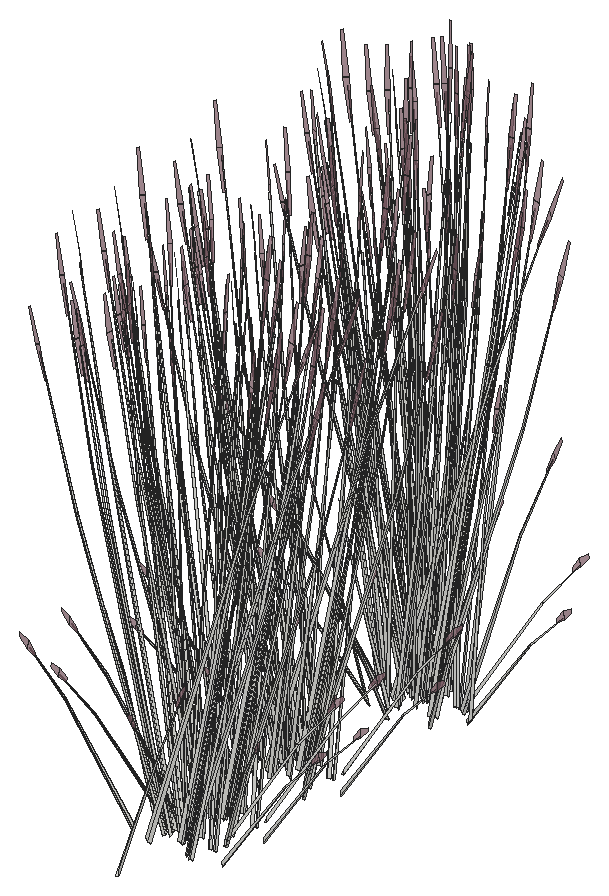
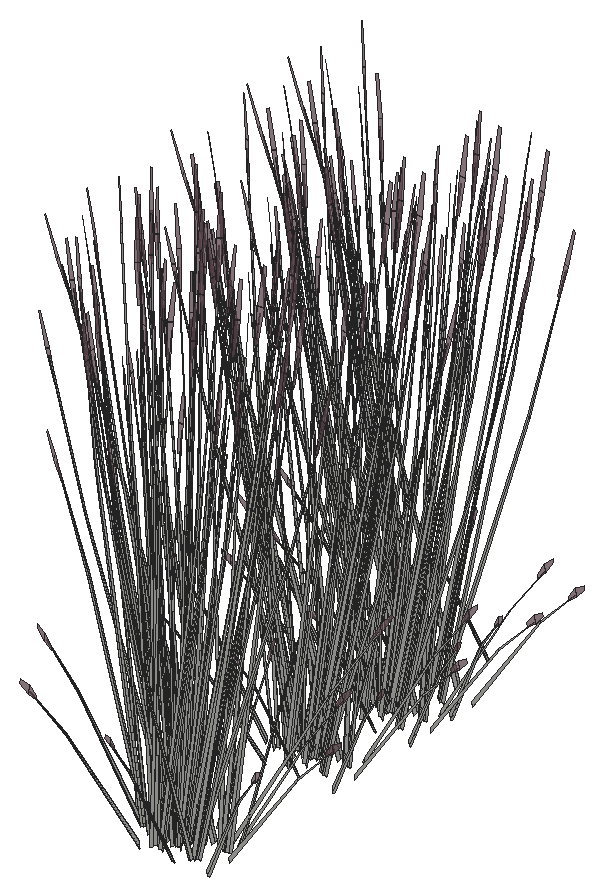
# SketchUp Ruby script. Lengths in inches.
U = 1.inch
M = Sketchup.active_model
def pt(a) = Geom::Point3d.new(a.map { |v| v * U })
def face(e, loops, mat)
  f = e.add_face(loops[0].map { |a| pt(a) })
  loops[1..].each { |l| e.add_face(l.map { |a| pt(a) }).erase! }
  f.material = f.back_material = mat if mat
  f
end
# faces: each face lists its corners as indices into pts; further lists are holes
def faces(e, pts, list, mat = nil) = list.each { |f| face(e, (f[0].is_a?(Array) ? f : [f]).map { |l| l.map { |i| pts[i] } }, mat) }
# xy, xz, yz: faces in a plane at the given z, y or x. An outline is a flat list of corners, or four numbers for a rectangle; further outlines are holes
def ring(l) = l.size == 4 ? [[l[0], l[1]], [l[2], l[1]], [l[2], l[3]], [l[0], l[3]]] : l.each_slice(2).to_a
def flat(e, list, mat, &to3) = list.each { |f| face(e, (f[0].is_a?(Array) ? f : [f]).map { |l| ring(l).map { |u, v| to3.(u, v) } }, mat) }
def xy(e, z, list, mat = nil) = flat(e, list, mat) { |x, y| [x, y, z] }
def xz(e, y, list, mat = nil) = flat(e, list, mat) { |x, z| [x, y, z] }
def yz(e, x, list, mat = nil) = flat(e, list, mat) { |y, z| [x, y, z] }
def lines(e, pts, list) = list.each { |a, b| e.add_line(pt(pts[a]), pt(pts[b])) }
# prism: a flat outline (further loops are holes) pulled along v
def prism(e, loops, v, mat = nil)
  f = face(e, loops, mat); d = Geom::Vector3d.new(v.map { |x| x * U })
  f.pushpull(f.normal.samedirection?(d) ? d.length : -d.length)
end
def box(e, o, s, mat = nil) = prism(e, [[o, [o[0] + s[0], o[1], o[2]], [o[0] + s[0], o[1] + s[1], o[2]], [o[0], o[1] + s[1], o[2]]]], [0, 0, s[2]], mat)
def at(x, y, z, deg = 0) = Geom::Transformation.translation(pt([x, y, z])) * Geom::Transformation.rotation(ORIGIN, Z_AXIS, deg.degrees)
def axes(o, x, y, z) = Geom::Transformation.new([*x, 0, *y, 0, *z, 0, *pt(o).to_a, 1])
def part(name) = M.definitions.add(name)
# library, detail: a bought-in or finely detailed component or shape, given as its bounding box
def library(name, o, s) = part(name).tap { |d| box(d.entities, o, s) }
def detail(e, o, s) = box(e.add_group.entities, o, s)
def put(e, d, t, mat = nil) = e.add_instance(d, t).tap { |i| i.material = mat if mat }
def group(e, t, mat = nil) = e.add_group.tap { |g| g.transformation = t; g.material = mat if mat }.entities
root = M.entities
M.materials.add("LightPink_Translucent").color = [144, 107, 117]
M.materials["LightPink_Translucent"].alpha = 0.75
c1 = part("blade")
p = [[2.15,0.21,22],[0,0.17,0],[0.09,0.45,0],[2.18,0.31,22],[2.29,0.31,22],[0.38,0.45,0],
  [2.48,0.24,33],[2.49,0.24,33],[2.48,0.22,33]]
faces(c1.entities,p,[[0,1,2,3],[4,5,2,3],[6,3,4,7],[8,0,3,6]])
c2 = part("seeds")
p = [[0.3,-0.1,1.38],[-0.01,-0.03,1.59],[-0.01,-0.03,0.03],[0.14,-0.07,-0.07],[0.29,-0.03,3],[0.15,0.01,3.11]]
faces(c2.entities,p,[[0,1,2,3],[1,0,4,5]],"LightPink_Translucent")
c3 = part("blade with seeds")
put(c3.entities,c1,at(0,0,0))
put(c3.entities,c2,axes([2.4,0.25,30.99],[1.5799,-0.05474,1.17369],[-0.12525,1.92788,0.29478],[-0.07173,-0.02425,1.56792]))
put(root,c3,axes([271.58,360.875,124.14],[0.14478,-0.0355,1.76342],[0.8709,0.19542,-0.26939],[0.02547,0.22025,0.30037]))
put(root,c3,axes([272.2,369.89,124.04],[-0.15005,0.02351,1.76342],[-0.82981,-0.26461,-0.26939],[0.01392,-0.22072,0.30037]))
put(root,c3,axes([271.59,368.48,124.89],[-0.53742,-0.54764,-0.44739],[0.81403,-0.38564,0.21531],[-0.17391,-0.06776,1.43643]))
put(root,c3,axes([271.11,368.69,124.73],[-0.9306,-0.10697,-0.62353],[0.19638,-0.65984,-0.16365],[-0.27771,-0.07995,1.37633]))
put(root,c3,axes([270.89,366.84,124.27],[-0.88056,0.26122,1.28929],[-0.28027,-0.74951,0.50096],[0.54072,0.01247,1.46642]))
put(root,c3,axes([277.77,367.86,124.17],[-0.04675,-0.09906,1.76342],[0.32428,-0.57943,-0.26939],[0.32711,-0.00833,0.30037]))
put(root,c3,axes([268.12,367.76,124.17],[0.02269,0.10283,1.76342],[-0.45738,0.53699,-0.26939],[-0.32488,-0.02707,0.30037]))
put(root,c3,axes([270.12,369.7,124.7],[-0.21015,-0.56852,-0.30978],[0.83462,-0.16144,0.30978],[-0.16826,-0.06556,1.38974]))
put(root,c3,axes([269.52,370.7,124.04],[-0.08666,0.08595,1.76342],[-0.87574,0.18531,-0.26939],[-0.21156,-0.16858,0.30037]))
put(root,c3,axes([273.17,367.23,125.34],[0.90324,-0.43318,-0.29095],[0.60064,0.61207,-0.50002],[0.22285,0.06216,1.59708]))
put(root,c3,axes([270.97,373.06,124.65],[-0.36739,-0.66907,-0.69835],[1.05831,-0.24096,-0.18329],[-0.04061,-0.22656,1.54149]))
put(root,c3,axes([275.88,371.01,124.04],[-0.1339,-0.0514,1.76342],[-0.34394,-0.57425,-0.26939],[0.23202,-0.15583,0.30037]))
put(root,c3,axes([269.89,369.94,124.69],[-0.83726,-0.32623,-0.49651],[0.50045,-0.58498,0],[-0.19069,-0.0743,1.57504]))
put(root,c3,axes([275.45,366.08,124.69],[0.83726,0.32623,-0.49651],[-0.50045,0.58498,0],[0.19069,0.0743,1.57504]))
put(root,c3,axes([272.17,368.79,125.34],[-0.90324,0.43318,-0.29095],[-0.60064,-0.61207,-0.50002],[-0.22285,-0.06216,1.59708]))
put(root,c3,axes([275.22,366.32,124.7],[0.21015,0.56852,-0.30978],[-0.83462,0.16144,0.30978],[0.16826,0.06556,1.38974]))
put(root,c3,axes([273.73,369.43,124.86],[0.93921,-0.22138,-0.19198],[0.33003,0.6377,0.00008],[0.10367,-0.02447,1.73897]))
put(root,c3,axes([274.23,367.33,124.73],[0.9306,0.10697,-0.62353],[-0.19638,0.65984,-0.16365],[0.27771,0.07995,1.37633]))
put(root,c3,axes([268.8,372.96,124.57],[0,-0.65246,-0.49651],[1.00089,0,0],[0,-0.1486,1.57504]))
put(root,c3,axes([271.58,371.03,124.57],[0.83726,-0.32623,-0.49651],[0.50045,0.58498,0],[0.19069,-0.0743,1.57504]))
put(root,c3,axes([272.57,372.37,124.61],[0.60257,-0.49041,-0.62353],[0.74854,0.44469,-0.16365],[0.24146,-0.12234,1.37633]))
put(root,c3,axes([273.75,367.54,124.89],[0.53742,0.54764,-0.44739],[-0.81403,0.38564,0.21531],[0.17391,0.06776,1.43643]))
put(root,c3,axes([271.53,373.23,124.76],[0.43405,-0.58792,-0.44739],[0.90188,0.28295,0.21531],[0,-0.13553,1.43643]))
put(root,c3,axes([272.74,368.875,124.89],[-0.97146,0.04028,-0.44739],[-0.08785,-0.66859,0.21531],[-0.17391,0.06776,1.43643]))
put(root,c3,axes([271.92,372.9375,125.21],[-0.10425,-0.7445,-0.29095],[1.08575,-0.04502,-0.50002],[0.19119,-0.09917,1.59708]))
put(root,c3,axes([269.23,372.98,124.58],[0.62448,-0.40708,-0.30978],[0.62448,0.40708,0.30978],[0,-0.13112,1.38974]))
put(root,c3,axes([271.42,373.72,125.21],[-1.00749,-0.31132,-0.29095],[0.48511,-0.65709,-0.50002],[-0.03166,-0.16133,1.59708]))
put(root,c3,axes([271.78,371.29,124.58],[0.83462,0.16144,-0.30978],[-0.21015,0.56852,0.30978],[0.16826,-0.06556,1.38974]))
put(root,c3,axes([273.5625,370.34,124.7],[-0.83462,-0.16144,-0.30978],[0.21015,-0.56852,0.30978],[-0.16826,0.06556,1.38974]))
put(root,c3,axes([271.67,374.41,124.99],[0.23711,-0.77313,-0.23429],[1.12425,0.13477,0.51271],[-0.19645,-0.10677,1.5644]))
put(root,c3,axes([273.92,367.91,125.34],[1.00749,0.31132,-0.29095],[-0.48511,0.65709,-0.50002],[0.03166,0.16133,1.59708]))
put(root,c3,axes([276.11,368.65,124.7],[-0.62448,0.40708,-0.30978],[-0.62448,-0.40708,0.30978],[0,0.13112,1.38974]))
put(root,c3,axes([273.42,368.69,125.34],[0.10425,0.7445,-0.29095],[-1.08575,0.04502,-0.50002],[-0.19119,0.09917,1.59708]))
put(root,c3,axes([273.81,368.4,124.89],[-0.43405,0.58792,-0.44739],[-0.90188,-0.28295,0.21531],[0,0.13553,1.43643]))
put(root,c3,axes([271.59,374.1,124.76],[-0.53742,-0.54764,-0.44739],[0.81403,-0.38564,0.21531],[-0.17391,-0.06776,1.43643]))
put(root,c3,axes([272.77,369.26,124.73],[-0.60257,0.49041,-0.62353],[-0.74854,-0.44469,-0.16365],[-0.24146,0.12234,1.37633]))
put(root,c3,axes([273.76,370.6,124.69],[-0.83726,0.32623,-0.49651],[-0.50045,-0.58498,0],[-0.19069,0.0743,1.57504]))
put(root,c3,axes([276.54,368.67,124.69],[0,0.65246,-0.49651],[-1.00089,0,0],[0,0.1486,1.57504]))
put(root,c3,axes([271.11,374.31,124.61],[-0.9306,-0.10697,-0.62353],[0.19638,-0.65984,-0.16365],[-0.27771,-0.07995,1.37633]))
put(root,c3,axes([270.89,372.46,124.14],[-0.88056,0.26122,1.28929],[-0.28027,-0.74951,0.50096],[0.54072,0.01247,1.46642]))
put(root,c3,axes([277.77,373.47,124.04],[-0.04675,-0.09906,1.76342],[0.32428,-0.57943,-0.26939],[0.32711,-0.00833,0.30037]))
put(root,c3,axes([275.41,370.72,124.17],[0.06518,-0.0942,1.76342],[0.82057,-0.27742,-0.26939],[0.24877,0.14358,0.30037]))
put(root,c3,axes([268.12,373.375,124.04],[0.02269,0.10283,1.76342],[-0.45738,0.53699,-0.26939],[-0.32488,-0.02707,0.30037]))
put(root,c3,axes([274.33,368.58,124.77],[0.32803,0.59738,-0.69212],[-0.94492,0.21515,-0.18165],[0.03626,0.20229,1.52773]))
put(root,c3,axes([267.875,370.64,124.17],[0.12,0.06519,1.76342],[0.20347,0.60397,-0.26939],[-0.26596,0.12879,0.30037]))
put(root,c3,axes([270.12,375.3125,124.58],[-0.21015,-0.56852,-0.30978],[0.83462,-0.16144,0.30978],[-0.16826,-0.06556,1.38974]))
put(root,c3,axes([273.17,372.84,125.21],[0.90324,-0.43318,-0.29095],[0.60064,0.61207,-0.50002],[0.22285,0.06216,1.59708]))
put(root,c3,axes([269.89,375.55,124.57],[-0.83726,-0.32623,-0.49651],[0.50045,-0.58498,0],[-0.19069,-0.0743,1.57504]))
put(root,c3,axes([275.45,371.69,124.57],[0.83726,0.32623,-0.49651],[-0.50045,0.58498,0],[0.19069,0.0743,1.57504]))
put(root,c3,axes([272.17,374.4,125.21],[-0.90324,0.43318,-0.29095],[-0.60064,-0.61207,-0.50002],[-0.22285,-0.06216,1.59708]))
put(root,c3,axes([275.22,371.94,124.58],[0.21015,0.56852,-0.30978],[-0.83462,0.16144,0.30978],[0.16826,0.06556,1.38974]))
put(root,c3,axes([273.73,375.05,124.73],[0.93921,-0.22138,-0.19198],[0.33003,0.6377,0.00008],[0.10367,-0.02447,1.73897]))
put(root,c3,axes([271.58,370.7,124.17],[0.14478,-0.0355,1.76342],[0.8709,0.19542,-0.26939],[0.02547,0.22025,0.30037]))
put(root,c3,axes([274.23,372.94,124.61],[0.9306,0.10697,-0.62353],[-0.19638,0.65984,-0.16365],[0.27771,0.07995,1.37633]))
put(root,c3,axes([273.18,374.6,125.01],[-0.87356,-0.52515,-0.25192],[0.73507,-0.5897,0.5513],[-0.23523,0.06143,1.68216]))
put(root,c3,axes([273.75,373.15,124.76],[0.53742,0.54764,-0.44739],[-0.81403,0.38564,0.21531],[0.17391,0.06776,1.43643]))
put(root,c3,axes([272.74,374.49,124.76],[-0.97146,0.04028,-0.44739],[-0.08785,-0.66859,0.21531],[-0.17391,0.06776,1.43643]))
put(root,c3,axes([272.2,380.25,124.07],[-0.15005,0.02351,1.76342],[-0.82981,-0.26461,-0.26939],[0.01392,-0.22072,0.30037]))
put(root,c3,axes([273.5625,375.96,124.58],[-0.83462,-0.16144,-0.30978],[0.21015,-0.56852,0.30978],[-0.16826,0.06556,1.38974]))
put(root,c3,axes([273.92,373.53,125.21],[1.00749,0.31132,-0.29095],[-0.48511,0.65709,-0.50002],[0.03166,0.16133,1.59708]))
put(root,c3,axes([276.11,374.27,124.58],[-0.62448,0.40708,-0.30978],[-0.62448,-0.40708,0.30978],[0,0.13112,1.38974]))
put(root,c3,axes([273.42,374.31,125.21],[0.10425,0.7445,-0.29095],[-1.08575,0.04502,-0.50002],[-0.19119,0.09917,1.59708]))
put(root,c3,axes([273.81,374.02,124.76],[-0.43405,0.58792,-0.44739],[-0.90188,-0.28295,0.21531],[0,0.13553,1.43643]))
put(root,c3,axes([272.77,374.875,124.61],[-0.60257,0.49041,-0.62353],[-0.74854,-0.44469,-0.16365],[-0.24146,0.12234,1.37633]))
put(root,c3,axes([273.76,376.21,124.57],[-0.83726,0.32623,-0.49651],[-0.50045,-0.58498,0],[-0.19069,0.0743,1.57504]))
put(root,c3,axes([276.54,374.28,124.57],[0,0.65246,-0.49651],[-1.00089,0,0],[0,0.1486,1.57504]))
put(root,c3,axes([269.52,381.06,124.07],[-0.08666,0.08595,1.76342],[-0.87574,0.18531,-0.26939],[-0.21156,-0.16858,0.30037]))
put(root,c3,axes([270.97,383.42,124.68],[-0.36739,-0.66907,-0.69835],[1.05831,-0.24096,-0.18329],[-0.04061,-0.22656,1.54149]))
put(root,c3,axes([275.88,381.375,124.07],[-0.1339,-0.0514,1.76342],[-0.34394,-0.57425,-0.26939],[0.23202,-0.15583,0.30037]))
put(root,c3,axes([275.41,376.33,124.04],[0.06518,-0.0942,1.76342],[0.82057,-0.27742,-0.26939],[0.24877,0.14358,0.30037]))
put(root,c3,axes([274.33,374.19,124.64],[0.32803,0.59738,-0.69212],[-0.94492,0.21515,-0.18165],[0.03626,0.20229,1.52773]))
put(root,c3,axes([267.875,376.25,124.04],[0.12,0.06519,1.76342],[0.20347,0.60397,-0.26939],[-0.26596,0.12879,0.30037]))
put(root,c3,axes([268.8,383.33,124.6],[0,-0.65246,-0.49651],[1.00089,0,0],[0,-0.1486,1.57504]))
put(root,c3,axes([271.58,381.39,124.6],[0.83726,-0.32623,-0.49651],[0.50045,0.58498,0],[0.19069,-0.0743,1.57504]))
put(root,c3,axes([272.57,382.73,124.64],[0.60257,-0.49041,-0.62353],[0.74854,0.44469,-0.16365],[0.24146,-0.12234,1.37633]))
put(root,c3,axes([271.58,376.3125,124.04],[0.14478,-0.0355,1.76342],[0.8709,0.19542,-0.26939],[0.02547,0.22025,0.30037]))
put(root,c3,axes([271.53,383.59,124.79],[0.43405,-0.58792,-0.44739],[0.90188,0.28295,0.21531],[0,-0.13553,1.43643]))
put(root,c3,axes([271.92,383.3,125.25],[-0.10425,-0.7445,-0.29095],[1.08575,-0.04502,-0.50002],[0.19119,-0.09917,1.59708]))
put(root,c3,axes([269.23,383.34,124.61],[0.62448,-0.40708,-0.30978],[0.62448,0.40708,0.30978],[0,-0.13112,1.38974]))
put(root,c3,axes([271.42,384.08,125.25],[-1.00749,-0.31132,-0.29095],[0.48511,-0.65709,-0.50002],[-0.03166,-0.16133,1.59708]))
put(root,c3,axes([271.78,381.65,124.61],[0.83462,0.16144,-0.30978],[-0.21015,0.56852,0.30978],[0.16826,-0.06556,1.38974]))
put(root,c3,axes([271.67,384.77,125.02],[0.23711,-0.77313,-0.23429],[1.12425,0.13477,0.51271],[-0.19645,-0.10677,1.5644]))
put(root,c3,axes([271.59,384.46,124.79],[-0.53742,-0.54764,-0.44739],[0.81403,-0.38564,0.21531],[-0.17391,-0.06776,1.43643]))
put(root,c3,axes([271.11,384.67,124.64],[-0.9306,-0.10697,-0.62353],[0.19638,-0.65984,-0.16365],[-0.27771,-0.07995,1.37633]))
put(root,c3,axes([270.89,382.82,124.17],[-0.88056,0.26122,1.28929],[-0.28027,-0.74951,0.50096],[0.54072,0.01247,1.46642]))
put(root,c3,axes([277.77,383.84,124.07],[-0.04675,-0.09906,1.76342],[0.32428,-0.57943,-0.26939],[0.32711,-0.00833,0.30037]))
put(root,c3,axes([268.12,383.74,124.07],[0.02269,0.10283,1.76342],[-0.45738,0.53699,-0.26939],[-0.32488,-0.02707,0.30037]))
put(root,c3,axes([270.12,385.67,124.61],[-0.21015,-0.56852,-0.30978],[0.83462,-0.16144,0.30978],[-0.16826,-0.06556,1.38974]))
put(root,c3,axes([273.17,383.21,125.25],[0.90324,-0.43318,-0.29095],[0.60064,0.61207,-0.50002],[0.22285,0.06216,1.59708]))
put(root,c3,axes([269.89,385.92,124.6],[-0.83726,-0.32623,-0.49651],[0.50045,-0.58498,0],[-0.19069,-0.0743,1.57504]))
put(root,c3,axes([275.45,382.05,124.6],[0.83726,0.32623,-0.49651],[-0.50045,0.58498,0],[0.19069,0.0743,1.57504]))
put(root,c3,axes([272.17,384.77,125.25],[-0.90324,0.43318,-0.29095],[-0.60064,-0.61207,-0.50002],[-0.22285,-0.06216,1.59708]))
put(root,c3,axes([275.22,382.3,124.61],[0.21015,0.56852,-0.30978],[-0.83462,0.16144,0.30978],[0.16826,0.06556,1.38974]))
put(root,c3,axes([273.73,385.41,124.77],[0.93921,-0.22138,-0.19198],[0.33003,0.6377,0.00008],[0.10367,-0.02447,1.73897]))
put(root,c3,axes([274.23,383.3,124.64],[0.9306,0.10697,-0.62353],[-0.19638,0.65984,-0.16365],[0.27771,0.07995,1.37633]))
put(root,c3,axes([273.18,384.96,125.05],[-0.87356,-0.52515,-0.25192],[0.73507,-0.5897,0.5513],[-0.23523,0.06143,1.68216]))
put(root,c3,axes([273.75,383.51,124.79],[0.53742,0.54764,-0.44739],[-0.81403,0.38564,0.21531],[0.17391,0.06776,1.43643]))
put(root,c3,axes([272.74,384.85,124.79],[-0.97146,0.04028,-0.44739],[-0.08785,-0.66859,0.21531],[-0.17391,0.06776,1.43643]))
put(root,c3,axes([273.5625,386.32,124.61],[-0.83462,-0.16144,-0.30978],[0.21015,-0.56852,0.30978],[-0.16826,0.06556,1.38974]))
put(root,c3,axes([273.92,383.89,125.25],[1.00749,0.31132,-0.29095],[-0.48511,0.65709,-0.50002],[0.03166,0.16133,1.59708]))
put(root,c3,axes([276.11,384.63,124.61],[-0.62448,0.40708,-0.30978],[-0.62448,-0.40708,0.30978],[0,0.13112,1.38974]))
put(root,c3,axes([273.42,384.67,125.25],[0.10425,0.7445,-0.29095],[-1.08575,0.04502,-0.50002],[-0.19119,0.09917,1.59708]))
put(root,c3,axes([273.81,384.38,124.79],[-0.43405,0.58792,-0.44739],[-0.90188,-0.28295,0.21531],[0,0.13553,1.43643]))
put(root,c3,axes([272.77,385.24,124.64],[-0.60257,0.49041,-0.62353],[-0.74854,-0.44469,-0.16365],[-0.24146,0.12234,1.37633]))
put(root,c3,axes([273.76,386.58,124.6],[-0.83726,0.32623,-0.49651],[-0.50045,-0.58498,0],[-0.19069,0.0743,1.57504]))
put(root,c3,axes([276.54,384.64,124.6],[0,0.65246,-0.49651],[-1.00089,0,0],[0,0.1486,1.57504]))
put(root,c3,axes([275.41,386.7,124.07],[0.06518,-0.0942,1.76342],[0.82057,-0.27742,-0.26939],[0.24877,0.14358,0.30037]))
put(root,c3,axes([274.33,384.56,124.68],[0.32803,0.59738,-0.69212],[-0.94492,0.21515,-0.18165],[0.03626,0.20229,1.52773]))
put(root,c3,axes([267.875,386.62,124.07],[0.12,0.06519,1.76342],[0.20347,0.60397,-0.26939],[-0.26596,0.12879,0.30037]))
put(root,c3,axes([271.58,386.67,124.07],[0.14478,-0.0355,1.76342],[0.8709,0.19542,-0.26939],[0.02547,0.22025,0.30037]))
put(root,c3,axes([272.2,397.36,123.41],[-0.15005,0.02351,1.76342],[-0.82981,-0.26461,-0.26939],[0.01392,-0.22072,0.30037]))
put(root,c3,axes([269.52,398.17,123.41],[-0.08666,0.08595,1.76342],[-0.87574,0.18531,-0.26939],[-0.21156,-0.16858,0.30037]))
put(root,c3,axes([270.97,400.53,124.01],[-0.36739,-0.66907,-0.69835],[1.05831,-0.24096,-0.18329],[-0.04061,-0.22656,1.54149]))
put(root,c3,axes([275.88,398.49,123.41],[-0.1339,-0.0514,1.76342],[-0.34394,-0.57425,-0.26939],[0.23202,-0.15583,0.30037]))
put(root,c3,axes([270.82,398.61,124.29],[-0.55932,-0.6538,0],[0.93577,-0.36461,-0.51607],[0.21313,-0.08304,1.63711]))
put(root,c3,axes([272.05,397.82,124.04],[-0.61821,0.37431,-0.03893],[-0.56645,-0.40995,-0.17649],[-0.03988,-0.11616,0.58215]))
put(root,c3,axes([268.8,400.4375,123.93],[0,-0.65246,-0.49651],[1.00089,0,0],[0,-0.1486,1.57504]))
put(root,c3,axes([271.58,398.51,123.93],[0.83726,-0.32623,-0.49651],[0.50045,0.58498,0],[0.19069,-0.0743,1.57504]))
put(root,c3,axes([272.57,399.84,123.97],[0.60257,-0.49041,-0.62353],[0.74854,0.44469,-0.16365],[0.24146,-0.12234,1.37633]))
put(root,c3,axes([271.53,400.7,124.125],[0.43405,-0.58792,-0.44739],[0.90188,0.28295,0.21531],[0,-0.13553,1.43643]))
put(root,c3,axes([271.92,400.41,124.58],[-0.10425,-0.7445,-0.29095],[1.08575,-0.04502,-0.50002],[0.19119,-0.09917,1.59708]))
put(root,c3,axes([269.23,400.45,123.94],[0.62448,-0.40708,-0.30978],[0.62448,0.40708,0.30978],[0,-0.13112,1.38974]))
put(root,c3,axes([268.98,398.5,124.04],[-0.25807,0.53277,-0.03893],[-0.79428,-0.16389,-0.17649],[-0.1206,-0.08714,0.58215]))
put(root,c3,axes([271.42,401.19,124.58],[-1.00749,-0.31132,-0.29095],[0.48511,-0.65709,-0.50002],[-0.03166,-0.16133,1.59708]))
put(root,c3,axes([268.55,400.93,124.29],[-1.11865,0,0],[0,-0.72922,-0.51607],[0,-0.16609,1.63711]))
put(root,c3,axes([268.74,399.63,124.51],[0.17466,0.18165,1.43002],[-0.40248,0.49377,-0.30754],[-0.41327,-0.11802,0.61141]))
put(root,c3,axes([271.78,398.76,123.94],[0.83462,0.16144,-0.30978],[-0.21015,0.56852,0.30978],[0.16826,-0.06556,1.38974]))
put(root,c3,axes([269.42,400.74,124.24],[-0.83213,0.54855,0.30756],[-0.83263,-0.54278,-0.36492],[-0.02906,-0.15578,1.64885]))
put(root,c3,axes([272.0625,401,124.35],[1.00799,0.31623,0.24065],[-0.48511,0.65709,0.50002],[0,-0.15147,1.60543]))
put(root,c3,axes([271.67,401.88,124.35],[0.23711,-0.77313,-0.23429],[1.12425,0.13477,0.51271],[-0.19645,-0.10677,1.5644]))
put(root,c3,axes([274.94,398.77,124.29],[0.55932,-0.6538,0],[0.93577,0.36461,-0.51607],[0.21313,0.08304,1.63711]))
put(root,c3,axes([271.59,401.57,124.125],[-0.53742,-0.54764,-0.44739],[0.81403,-0.38564,0.21531],[-0.17391,-0.06776,1.43643]))
put(root,c3,axes([271.7,400.8,124.28],[0.38895,0.72959,0.45755],[-1.11135,0.2537,0.17955],[0.01358,-0.13406,1.58856]))
put(root,c3,axes([277.14,401.36,123.9],[-0.57619,0.0783,1.41583],[-0.09171,-0.62326,0.08104],[0.40356,-0.09434,0.80566]))
put(root,c3,axes([278.19,400.8,124.18],[-0.55463,-0.41721,-0.06488],[0.60744,-0.38228,-0.29416],[0.17212,-0.02691,0.97024]))
put(root,c3,axes([273.1,400.86,124.12],[0,-0.75495,0],[1.11865,0,0],[0,0,1.79456]))
put(root,c3,axes([271.11,401.78,123.97],[-0.9306,-0.10697,-0.62353],[0.19638,-0.65984,-0.16365],[-0.27771,-0.07995,1.37633]))
put(root,c3,axes([272.57,400.38,124.28],[-0.74176,0.59212,0.45755],[-0.88124,-0.52269,0.17955],[0.17882,-0.05909,1.58856]))
put(root,c3,axes([273.38,401.44,124.21],[-0.83213,-0.56158,-0.06131],[0.83263,-0.56193,0],[-0.02906,-0.01961,1.75571]))
put(root,c3,axes([270.89,399.93,123.51],[-0.88056,0.26122,1.28929],[-0.28027,-0.74951,0.50096],[0.54072,0.01247,1.46642]))
put(root,c3,axes([273.26,400.13,124.53],[0.17258,-0.58229,0.1448],[0.84319,0.10108,-0.41347],[0.15345,0.05979,1.26744]))
put(root,c3,axes([271.8,401.51,124.28],[1.13071,0.13747,0.45755],[-0.23011,0.77639,0.17955],[-0.16524,-0.07497,1.58856]))
put(root,c3,axes([277.77,400.95,123.41],[-0.04675,-0.09906,1.76342],[0.32428,-0.57943,-0.26939],[0.32711,-0.00833,0.30037]))
put(root,c3,axes([268.12,400.85,123.41],[0.02269,0.10283,1.76342],[-0.45738,0.53699,-0.26939],[-0.32488,-0.02707,0.30037]))
put(root,c3,axes([270.12,402.79,123.94],[-0.21015,-0.56852,-0.30978],[0.83462,-0.16144,0.30978],[-0.16826,-0.06556,1.38974]))
put(root,c3,axes([273.17,400.32,124.58],[0.90324,-0.43318,-0.29095],[0.60064,0.61207,-0.50002],[0.22285,0.06216,1.59708]))
put(root,c3,axes([269.89,403.03,123.93],[-0.83726,-0.32623,-0.49651],[0.50045,-0.58498,0],[-0.19069,-0.0743,1.57504]))
put(root,c3,axes([275.45,399.17,123.93],[0.83726,0.32623,-0.49651],[-0.50045,0.58498,0],[0.19069,0.0743,1.57504]))
put(root,c3,axes([273.86,401.03,124.12],[1.00089,0,0],[0,0.67548,0],[0,0,1.78407]))
put(root,c3,axes([272.17,401.88,124.58],[-0.90324,0.43318,-0.29095],[-0.60064,-0.61207,-0.50002],[-0.22285,-0.06216,1.59708]))
put(root,c3,axes([275.22,399.41,123.94],[0.21015,0.56852,-0.30978],[-0.83462,0.16144,0.30978],[0.16826,0.06556,1.38974]))
put(root,c3,axes([273.54,400.68,124.3],[-1.13071,-0.13747,0.49198],[0.23011,-0.77639,0.19306],[0.16524,0.07497,1.70813]))
put(root,c3,axes([272.64,402.6,124.12],[-0.29189,-0.56252,0],[0.83351,-0.19699,0],[0,0,1.54371]))
put(root,c3,axes([272.08,402.07,124.53],[-0.17258,0.58229,0.1448],[-0.84319,-0.10108,-0.41347],[-0.15345,-0.05979,1.26744]))
put(root,c3,axes([273.73,402.52,124.1],[0.93921,-0.22138,-0.19198],[0.33003,0.6377,0.00008],[0.10367,-0.02447,1.73897]))
put(root,c3,axes([273.84,401.32,124.13],[0.62448,0.42144,0],[-0.62448,0.42144,0],[0,0,1.69266]))
put(root,c3,axes([274.23,400.42,123.97],[0.9306,0.10697,-0.62353],[-0.19638,0.65984,-0.16365],[0.27771,0.07995,1.37633]))
put(root,c3,axes([272.43,402.85,124.11],[-0.90188,-0.29293,0],[0.43405,-0.60866,0],[0,0,1.62707]))
put(root,c3,axes([273.18,402.07,124.38],[-0.87356,-0.52515,-0.25192],[0.73507,-0.5897,0.5513],[-0.23523,0.06143,1.68216]))
put(root,c3,axes([273.67,401.16,124.21],[0,0.75458,-0.05637],[-1.11865,0,0],[0,0.02371,1.79368]))
put(root,c3,axes([273.75,400.625,124.125],[0.53742,0.54764,-0.44739],[-0.81403,0.38564,0.21531],[0.17391,0.06776,1.43643]))
put(root,c3,axes([270.4,403.42,124.29],[-0.55932,0.6538,0],[-0.93577,-0.36461,-0.51607],[-0.21313,-0.08304,1.63711]))
put(root,c3,axes([274.21,400.96,124.53],[0.83351,-0.19028,0.1448],[0.29189,0.54335,-0.41347],[0,0.11958,1.26744]))
put(root,c3,axes([272.74,401.96,124.125],[-0.97146,0.04028,-0.44739],[-0.08785,-0.66859,0.21531],[-0.17391,0.06776,1.43643]))
put(root,c3,axes([273.45,402.87,124.12],[0.90188,0.29293,0],[-0.43405,0.60866,0],[0,0,1.74954]))
put(root,c3,axes([273.8125,403.51,124.11],[-0.55235,-0.65609,-0.05142],[0.93577,-0.36461,0.51607],[-0.23059,0.06247,1.6363]))
put(root,c3,axes([273.62,401.93,124.53],[0.66093,0.39201,0.1448],[-0.5513,0.44227,-0.41347],[-0.15345,0.05979,1.26744]))
put(root,c3,axes([273.13,402.62,124.21],[0.38895,0.74956,-0.06012],[-1.11135,0.26265,0],[0.01358,0.02618,1.72173]))
put(root,c3,axes([273.5625,403.43,123.94],[-0.83462,-0.16144,-0.30978],[0.21015,-0.56852,0.30978],[-0.16826,0.06556,1.38974]))
put(root,c3,axes([276.79,401.26,124.29],[1.11865,0,0],[0,0.72922,-0.51607],[0,0.16609,1.63711]))
put(root,c3,axes([276.34,401.64,124.11],[-1.1181,-0.00522,-0.04976],[0,-0.72922,0.49943],[-0.03514,0.166,1.58352]))
put(root,c3,axes([273.92,401,124.58],[1.00749,0.31132,-0.29095],[-0.48511,0.65709,-0.50002],[0.03166,0.16133,1.59708]))
put(root,c3,axes([276.11,401.74,123.94],[-0.62448,0.40708,-0.30978],[-0.62448,-0.40708,0.30978],[0,0.13112,1.38974]))
put(root,c3,axes([273.42,401.78,124.58],[0.10425,0.7445,-0.29095],[-1.08575,0.04502,-0.50002],[-0.19119,0.09917,1.59708]))
put(root,c3,axes([273.81,401.49,124.125],[-0.43405,0.58792,-0.44739],[-0.90188,-0.28295,0.21531],[0,0.13553,1.43643]))
put(root,c3,axes([272.77,402.35,123.97],[-0.60257,0.49041,-0.62353],[-0.74854,-0.44469,-0.16365],[-0.24146,0.12234,1.37633]))
put(root,c3,axes([273.84,403.18,124.24],[1.11998,0.21207,0.30756],[-0.2802,0.75803,-0.36492],[-0.18537,0.09487,1.64885]))
put(root,c3,axes([273.76,403.6875,123.93],[-0.83726,0.32623,-0.49651],[-0.50045,-0.58498,0],[-0.19069,0.0743,1.57504]))
put(root,c3,axes([276.54,401.76,123.93],[0,0.65246,-0.49651],[-1.00089,0,0],[0,0.1486,1.57504]))
put(root,c3,axes([274.52,403.59,124.29],[0.55932,0.6538,0],[-0.93577,0.36461,-0.51607],[-0.21313,0.08304,1.63711]))
put(root,c3,axes([275.41,403.81,123.41],[0.06518,-0.0942,1.76342],[0.82057,-0.27742,-0.26939],[0.24877,0.14358,0.30037]))
put(root,c3,axes([274.33,401.67,124.01],[0.32803,0.59738,-0.69212],[-0.94492,0.21515,-0.18165],[0.03626,0.20229,1.52773]))
put(root,c3,axes([267.875,403.73,123.41],[0.12,0.06519,1.76342],[0.20347,0.60397,-0.26939],[-0.26596,0.12879,0.30037]))
put(root,c3,axes([271.58,403.79,123.41],[0.14478,-0.0355,1.76342],[0.8709,0.19542,-0.26939],[0.02547,0.22025,0.30037]))
put(root,c3,axes([269.57,403.875,124.74],[0.8127,-0.11554,0.06507],[0.18684,0.46549,-0.86304],[-0.05152,0.23564,0.7736]))
